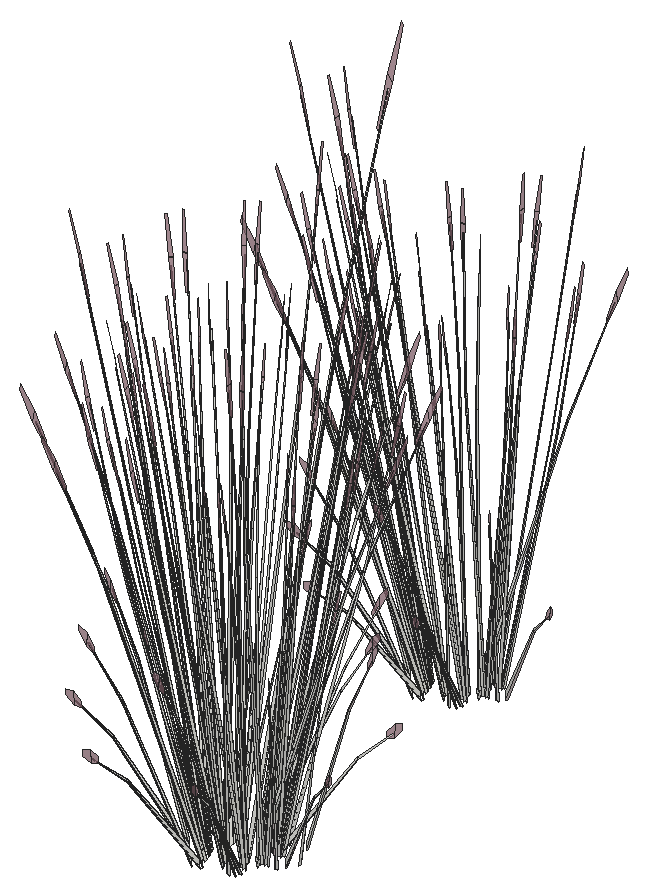
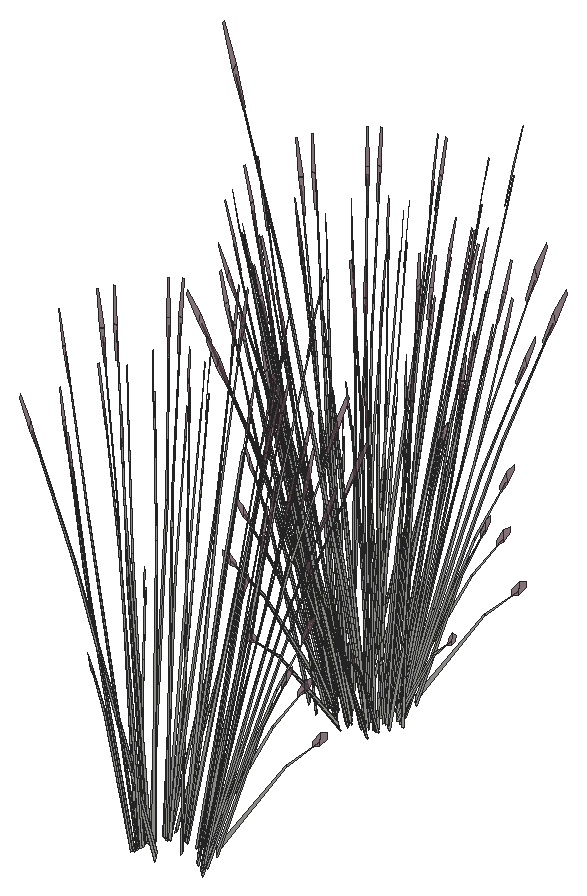
# SketchUp Ruby script. Lengths in inches.
U = 1.inch
M = Sketchup.active_model
def pt(a) = Geom::Point3d.new(a.map { |v| v * U })
def face(e, loops, mat)
  f = e.add_face(loops[0].map { |a| pt(a) })
  loops[1..].each { |l| e.add_face(l.map { |a| pt(a) }).erase! }
  f.material = f.back_material = mat if mat
  f
end
# faces: each face lists its corners as indices into pts; further lists are holes
def faces(e, pts, list, mat = nil) = list.each { |f| face(e, (f[0].is_a?(Array) ? f : [f]).map { |l| l.map { |i| pts[i] } }, mat) }
# xy, xz, yz: faces in a plane at the given z, y or x. An outline is a flat list of corners, or four numbers for a rectangle; further outlines are holes
def ring(l) = l.size == 4 ? [[l[0], l[1]], [l[2], l[1]], [l[2], l[3]], [l[0], l[3]]] : l.each_slice(2).to_a
def flat(e, list, mat, &to3) = list.each { |f| face(e, (f[0].is_a?(Array) ? f : [f]).map { |l| ring(l).map { |u, v| to3.(u, v) } }, mat) }
def xy(e, z, list, mat = nil) = flat(e, list, mat) { |x, y| [x, y, z] }
def xz(e, y, list, mat = nil) = flat(e, list, mat) { |x, z| [x, y, z] }
def yz(e, x, list, mat = nil) = flat(e, list, mat) { |y, z| [x, y, z] }
def lines(e, pts, list) = list.each { |a, b| e.add_line(pt(pts[a]), pt(pts[b])) }
# prism: a flat outline (further loops are holes) pulled along v
def prism(e, loops, v, mat = nil)
  f = face(e, loops, mat); d = Geom::Vector3d.new(v.map { |x| x * U })
  f.pushpull(f.normal.samedirection?(d) ? d.length : -d.length)
end
def box(e, o, s, mat = nil) = prism(e, [[o, [o[0] + s[0], o[1], o[2]], [o[0] + s[0], o[1] + s[1], o[2]], [o[0], o[1] + s[1], o[2]]]], [0, 0, s[2]], mat)
def at(x, y, z, deg = 0) = Geom::Transformation.translation(pt([x, y, z])) * Geom::Transformation.rotation(ORIGIN, Z_AXIS, deg.degrees)
def axes(o, x, y, z) = Geom::Transformation.new([*x, 0, *y, 0, *z, 0, *pt(o).to_a, 1])
def part(name) = M.definitions.add(name)
# library, detail: a bought-in or finely detailed component or shape, given as its bounding box
def library(name, o, s) = part(name).tap { |d| box(d.entities, o, s) }
def detail(e, o, s) = box(e.add_group.entities, o, s)
def put(e, d, t, mat = nil) = e.add_instance(d, t).tap { |i| i.material = mat if mat }
def group(e, t, mat = nil) = e.add_group.tap { |g| g.transformation = t; g.material = mat if mat }.entities
root = M.entities
M.materials.add("LightPink_Translucent").color = [144, 107, 117]
M.materials["LightPink_Translucent"].alpha = 0.75
c1 = part("blade")
p = [[2.15,0.21,22],[0,0.17,0],[0.09,0.45,0],[2.18,0.31,22],[2.29,0.31,22],[0.38,0.45,0],
  [2.48,0.24,33],[2.49,0.24,33],[2.48,0.22,33]]
faces(c1.entities,p,[[0,1,2,3],[4,5,2,3],[6,3,4,7],[8,0,3,6]])
c2 = part("seeds")
p = [[0.3,-0.1,1.38],[-0.01,-0.03,1.59],[-0.01,-0.03,0.03],[0.14,-0.07,-0.07],[0.29,-0.03,3],[0.15,0.01,3.11]]
faces(c2.entities,p,[[0,1,2,3],[1,0,4,5]],"LightPink_Translucent")
c3 = part("blade with seeds")
put(c3.entities,c1,at(0,0,0))
put(c3.entities,c2,axes([2.4,0.25,30.99],[1.5799,-0.05474,1.17369],[-0.12525,1.92788,0.29478],[-0.07173,-0.02425,1.56792]))
put(root,c3,axes([301.2,192.59,150.27],[0.09368,0.15143,1.44779],[-0.43286,0.12749,0.11706],[-0.09783,-0.23774,0.61892]))
put(root,c3,axes([301.91,191.58,150.98],[-0.06268,-0.06613,1.47793],[-0.4183,0.04193,-0.23373],[-0.06676,-0.15817,0.11853]))
put(root,c3,axes([303.79,192.39,150.98],[-0.00396,-0.09387,1.47793],[-0.33411,-0.2713,-0.23373],[0.05166,-0.16446,0.11853]))
put(root,c3,axes([302.39,192.375,150.82],[0.12355,-0.36271,-0.29918],[0.36044,0.10579,0.38624],[-0.03305,-0.14603,0.73904]))
put(root,c3,axes([302.66,192.85,150.27],[-0.0763,0.16212,1.44779],[-0.3201,-0.3355,0.11706],[0.1444,-0.2091,0.61892]))
put(root,c3,axes([303.7,192.06,150.98],[-0.04162,0.03603,1.49853],[-0.40776,-0.12155,-0.1416],[-0.01476,-0.15722,0.26519]))
put(root,c3,axes([301.49,191.37,150.98],[-0.00765,0.05653,1.49853],[-0.37706,0.20517,-0.1416],[-0.11096,-0.10488,0.26519]))
put(root,c3,axes([302.43,192.46,151],[0.4038,0.12331,0.40553],[-0.13808,0.40538,0.33437],[-0.02427,-0.15942,0.83914]))
put(root,c3,axes([302.55,192.6,151.25],[-0.40102,0.2196,-0.10273],[-0.19707,-0.38974,-0.57019],[-0.05291,-0.16424,0.8664]))
put(root,c3,axes([303.38,193.1,151.25],[-0.45039,-0.02337,-0.10273],[0.01231,-0.44247,-0.57019],[0.03129,-0.17041,0.8664]))
put(root,c3,axes([303.35,192.8125,150.82],[0.27728,-0.24833,-0.29918],[0.26248,0.28355,0.38624],[0.03994,-0.14407,0.73904]))
put(root,c3,axes([302.54,192.43,151],[0.30197,-0.1603,0.05432],[0.1478,0.29231,0.42765],[-0.02916,-0.12885,0.65209]))
put(root,c3,axes([301.35,192.51,150.82],[-0.06329,-0.37991,-0.29918],[0.36182,-0.10032,0.38624],[-0.09718,-0.10887,0.73904]))
put(root,c3,axes([301.51,192.47,151],[0.18625,-0.29962,0.05432],[0.26523,0.17444,0.42765],[-0.08575,-0.09606,0.65209]))
put(root,c3,axes([300.57,193.06,150.27],[0.15222,0.08126,1.44779],[-0.31502,0.34091,0.11706],[-0.19634,-0.15379,0.61892]))
put(root,c3,axes([302.43,192.76,151.27],[-0.12355,0.36271,0.29918],[-0.36044,-0.10579,-0.38624],[-0.03305,-0.14603,0.73904]))
put(root,c3,axes([303.35,192.91,151],[0.29182,0.32181,0.40553],[-0.3099,0.27755,0.33437],[0.05383,-0.15098,0.83914]))
put(root,c3,axes([301.59,192.44,151.59],[-0.2735,0.45217,-0.11506],[-0.39608,-0.2605,-0.63862],[-0.13768,-0.12775,0.97037]))
put(root,c3,axes([303.46,192.9375,151],[0.33677,0.02198,0.05432],[-0.00923,0.33185,0.42765],[0.03524,-0.12712,0.65209]))
put(root,c3,axes([303.21,193.16,151.27],[-0.27728,0.24833,0.29918],[-0.26248,-0.28355,-0.38624],[0.03994,-0.14407,0.73904]))
put(root,c3,axes([300.54,192.31,150.98],[-0.08817,-0.00333,1.47793],[-0.28072,0.33293,-0.23373],[-0.14978,-0.06803,0.11853]))
put(root,c3,axes([303.875,193.97,151.25],[-0.37908,-0.26007,-0.10273],[0.21839,-0.37663,-0.57019],[0.1071,-0.13092,0.8664]))
put(root,c3,axes([301.56,192.82,151.27],[0.06329,0.37991,0.29918],[-0.36182,0.10032,-0.38624],[-0.09718,-0.10887,0.73904]))
put(root,c3,axes([304.81,193.85,150.98],[-0.05353,-0.00358,1.49853],[-0.22227,-0.38383,-0.1416],[0.08926,-0.1262,0.26519]))
put(root,c3,axes([303.98,193.7,150.82],[0.35672,-0.06741,-0.29918],[0.09419,0.38534,0.38624],[0.10222,-0.1035,0.73904]))
put(root,c3,axes([300.63,193.0625,151],[0.02064,-0.35866,0.05432],[0.3116,0.00983,0.42765],[-0.11936,-0.03753,0.65209]))
put(root,c3,axes([300.51,193.17,150.82],[-0.23317,-0.29531,-0.29918],[0.26625,-0.27955,0.38624],[-0.13527,-0.04253,0.73904]))
put(root,c3,axes([303.6875,193.93,151.27],[-0.35672,0.06741,0.29918],[-0.09419,-0.38534,-0.38624],[0.10222,-0.1035,0.73904]))
put(root,c3,axes([304.01,193.87,151],[0.28133,0.19836,0.05432],[-0.16379,0.28248,0.42765],[0.0902,-0.09132,0.65209]))
put(root,c3,axes([303.93,193.79,151],[0.10163,0.43409,0.40553],[-0.39868,0.07534,0.33437],[0.1175,-0.10209,0.83914]))
put(root,c3,axes([305.01,194.3125,150.98],[0.05687,-0.07184,1.47793],[-0.07279,-0.44069,-0.23373],[0.14268,-0.08356,0.11853]))
put(root,c3,axes([300.2,192.59,150.98],[0.03038,0.04707,1.49853],[-0.14646,0.42312,-0.1416],[-0.14833,0.00306,0.26519]))
put(root,c3,axes([300.84,193.33,151.27],[0.23317,0.29531,0.29918],[-0.26625,0.27955,-0.38624],[-0.13527,-0.04253,0.73904]))
put(root,c3,axes([300.78,193.14,151.25],[-0.02194,0.47967,-0.10273],[-0.41546,-0.01311,-0.57019],[-0.16001,-0.03332,0.8664]))
put(root,c3,axes([303.89,194.98,151.25],[-0.20619,-0.42709,-0.10273],[0.36595,-0.20988,-0.57019],[0.15422,-0.05635,0.8664]))
put(root,c3,axes([300.25,193.8,150.27],[0.16998,-0.01068,1.44779],[-0.11276,0.46299,0.11706],[-0.24224,-0.02864,0.61892]))
put(root,c3,axes([303.75,194.85,151.27],[-0.34057,-0.13158,0.29918],[0.09933,-0.38387,-0.38624],[0.13712,-0.0352,0.73904]))
put(root,c3,axes([300.18,194.15,151],[0.11578,-0.43006,0.40553],[0.38064,0.14706,0.33437],[-0.14969,0.02584,0.83914]))
put(root,c3,axes([300.15,194.04,151],[-0.15051,-0.3216,0.05432],[0.27447,-0.15741,0.42765],[-0.12099,0.03106,0.65209]))
put(root,c3,axes([304.1,194.8125,150.82],[0.34057,0.13158,-0.29918],[-0.09933,0.38387,0.38624],[0.13712,-0.0352,0.73904]))
put(root,c3,axes([300.1,194.2,150.82],[-0.34057,-0.13158,-0.29918],[0.09933,-0.38387,0.38624],[-0.13712,0.0352,0.73904]))
put(root,c3,axes([303.18,194.34,150.27],[-0.16998,0.01068,1.44779],[0.11276,-0.46299,0.11706],[0.24224,0.02864,0.61892]))
put(root,c3,axes([304.05,194.97,151],[0.15051,0.3216,0.05432],[-0.27447,0.15741,0.42765],[0.12099,-0.03106,0.65209]))
put(root,c3,axes([304.03,194.86,151],[-0.11578,0.43006,0.40553],[-0.38064,-0.14706,0.33437],[0.14969,-0.02584,0.83914]))
put(root,c3,axes([300.46,194.16,151.27],[0.34057,0.13158,0.29918],[-0.09933,0.38387,-0.38624],[-0.13712,0.0352,0.73904]))
put(root,c3,axes([304.71,196.25,150.98],[-0.03706,-0.04129,1.49853],[0.08106,-0.44261,-0.1416],[0.14596,-0.02828,0.26519]))
put(root,c3,axes([299.89,194.45,150.98],[-0.06692,0.06124,1.47793],[0.00569,0.44742,-0.23373],[-0.15339,0.05818,0.11853]))
put(root,c3,axes([300.32,194.03,151.25],[0.20619,0.42709,-0.10273],[-0.36595,0.20988,-0.57019],[-0.15422,0.05635,0.8664]))
put(root,c3,axes([304.39,195.88,150.32],[-0.07843,-0.39649,-0.0295],[0.37072,-0.09115,-0.13375],[0.07742,0.02514,0.44114]))
put(root,c3,axes([303.43,195.87,151.25],[0.02194,-0.47967,-0.10273],[0.41546,0.01311,-0.57019],[0.16001,0.03332,0.8664]))
put(root,c3,axes([303.36,195.68,151.27],[-0.23317,-0.29531,0.29918],[0.26625,-0.27955,-0.38624],[0.13527,0.04253,0.73904]))
put(root,c3,axes([303.79,195.58,150.98],[0.08791,-0.00798,1.47793],[0.24113,-0.36643,-0.23373],[0.15637,0.04837,0.11853]))
put(root,c3,axes([300.27,195.22,151],[-0.10163,-0.43409,0.40553],[0.39868,-0.07534,0.33437],[-0.1175,0.10209,0.83914]))
put(root,c3,axes([300.19,195.14,151],[-0.28133,-0.19836,0.05432],[0.16379,-0.28248,0.42765],[-0.0902,0.09132,0.65209]))
put(root,c3,axes([300.32,194.62,150.27],[0.14219,-0.09977,1.44779],[0.11971,0.461,0.11706],[-0.22323,0.10419,0.61892]))
put(root,c3,axes([300.52,195.08,151.27],[0.35672,-0.06741,0.29918],[0.09419,0.38534,-0.38624],[-0.10222,0.1035,0.73904]))
put(root,c3,axes([299.14,194.91,150.98],[0.0523,0.01265,1.49853],[0.16179,0.41674,-0.1416],[-0.10706,0.10938,0.26519]))
put(root,c3,axes([303.69,195.84,150.82],[0.23317,0.29531,-0.29918],[-0.26625,0.27955,0.38624],[0.13527,0.04253,0.73904]))
put(root,c3,axes([303.57,195.95,151],[-0.02064,0.35866,0.05432],[-0.3116,-0.00983,0.42765],[0.11936,0.03753,0.65209]))
put(root,c3,axes([300.23,195.31,150.82],[-0.35672,0.06741,-0.29918],[-0.09419,-0.38534,0.38624],[-0.10222,0.1035,0.73904]))
put(root,c3,axes([303.6,195.83,151],[-0.30217,0.31079,0.40553],[-0.2606,-0.33005,0.33437],[0.14177,0.05733,0.83914]))
put(root,c3,axes([302.64,196.19,151.27],[-0.06329,-0.37991,0.29918],[0.36182,-0.10032,-0.38624],[0.09718,0.10887,0.73904]))
put(root,c3,axes([302.86,195.08,150.27],[-0.15222,-0.08126,1.44779],[0.31502,-0.34091,0.11706],[0.19634,0.15379,0.61892]))
put(root,c3,axes([302.88,194.01,150.78],[-0.35411,-0.24507,1.16821],[0.37391,-0.38156,0.50405],[0.11425,0.22994,1.12919]))
put(root,c3,axes([300.33,195.04,151.25],[0.37908,0.26007,-0.10273],[-0.21839,0.37663,-0.57019],[-0.1071,0.13092,0.8664]))
put(root,c3,axes([302.61,196.39,151.25],[0.2442,-0.40372,-0.10273],[0.35364,0.23259,-0.57019],[0.12293,0.11406,0.8664]))
put(root,c3,axes([300.84,194.93,150.27],[0.10236,-0.14492,1.44779],[0.25844,0.39118,0.11706],[-0.17726,0.17814,0.61892]))
put(root,c3,axes([301,195.85,151.27],[0.27728,-0.24833,0.29918],[0.26248,0.28355,-0.38624],[-0.03994,0.14407,0.73904]))
put(root,c3,axes([302.29,196.73,150.98],[0.00121,-0.0571,1.49853],[0.35119,-0.25193,-0.1416],[0.12199,0.08992,0.26519]))
put(root,c3,axes([300.75,196.07,151],[-0.33677,-0.02198,0.05432],[0.00923,-0.33185,0.42765],[-0.03524,0.12712,0.65209]))
put(root,c3,axes([300.85,196.1,151],[-0.29182,-0.32181,0.40553],[0.3099,-0.27755,0.33437],[-0.05383,0.15098,0.83914]))
put(root,c3,axes([301.78,196.25,151.27],[0.12355,-0.36271,0.29918],[0.36044,0.10579,-0.38624],[0.03305,0.14603,0.73904]))
put(root,c3,axes([302.7,196.54,151],[-0.18625,0.29962,0.05432],[-0.26523,-0.17444,0.42765],[0.08575,0.09606,0.65209]))
put(root,c3,axes([302.78,196.45,151],[-0.4076,0.10824,0.40553],[-0.07074,-0.4246,0.33437],[0.09586,0.12514,0.83914]))
put(root,c3,axes([300.77,195.28,150.27],[0.0763,-0.16212,1.44779],[0.3201,0.3355,0.11706],[-0.1444,0.2091,0.61892]))
put(root,c3,axes([301.66,196.58,151],[-0.30197,0.1603,0.05432],[-0.1478,-0.29231,0.42765],[0.02916,0.12885,0.65209]))
put(root,c3,axes([300.85,196.2,150.82],[-0.27728,0.24833,-0.29918],[-0.26248,-0.28355,0.38624],[-0.03994,0.14407,0.73904]))
put(root,c3,axes([299.9,196.125,150.98],[-0.01019,0.09334,1.47793],[0.28908,0.3247,-0.23373],[-0.07568,0.15355,0.11853]))
put(root,c3,axes([300.82,195.91,151.56],[0.45039,0.02337,-0.11403],[-0.01231,0.44247,-0.63292],[-0.03129,0.17041,0.9617]))
put(root,c3,axes([301.66,196.41,151.25],[0.40102,-0.2196,-0.10273],[0.19707,0.38974,-0.57019],[0.05291,0.16424,0.8664]))
put(root,c3,axes([302.23,195.55,150.27],[-0.09368,-0.15143,1.44779],[0.43286,-0.12749,0.11706],[0.09783,0.23774,0.61892]))
put(root,c3,axes([301.82,196.64,150.82],[-0.12355,0.36271,-0.29918],[-0.36044,-0.10579,0.38624],[0.03305,0.14603,0.73904]))
put(root,c3,axes([299.87,197.08,150.98],[0.04649,-0.02848,1.49853],[0.38427,0.18941,-0.1416],[-0.00903,0.15771,0.26519]))
put(root,c3,axes([301.46,195.625,150.27],[-0.01003,-0.18103,1.44779],[0.43473,0.12009,0.11706],[-0.02689,0.25798,0.61892]))
put(root,c3,axes([301.5625,197.28,150.98],[0.05195,0.07595,1.47793],[0.41921,0.02984,-0.23373],[0.04216,0.1675,0.11853]))
put(root,c3,axes([299.2,211.99,150.27],[0.09368,0.15143,1.44779],[-0.43286,0.12749,0.11706],[-0.09783,-0.23774,0.61892]))
put(root,c3,axes([299.91,210.99,150.98],[-0.06268,-0.06613,1.47793],[-0.4183,0.04193,-0.23373],[-0.06676,-0.15817,0.11853]))
put(root,c3,axes([301.79,211.8,150.98],[-0.00396,-0.09387,1.47793],[-0.33411,-0.2713,-0.23373],[0.05166,-0.16446,0.11853]))
put(root,c3,axes([300.39,211.78,150.82],[0.12355,-0.36271,-0.29918],[0.36044,0.10579,0.38624],[-0.03305,-0.14603,0.73904]))
put(root,c3,axes([300.66,212.26,150.27],[-0.0763,0.16212,1.44779],[-0.3201,-0.3355,0.11706],[0.1444,-0.2091,0.61892]))
put(root,c3,axes([301.7,211.46,150.98],[-0.04162,0.03603,1.49853],[-0.40776,-0.12155,-0.1416],[-0.01476,-0.15722,0.26519]))
put(root,c3,axes([299.49,210.77,150.98],[-0.00765,0.05653,1.49853],[-0.37706,0.20517,-0.1416],[-0.11096,-0.10488,0.26519]))
put(root,c3,axes([300.43,211.87,151],[0.4038,0.12331,0.40553],[-0.13808,0.40538,0.33437],[-0.02427,-0.15942,0.83914]))
put(root,c3,axes([300.55,212.01,151.25],[-0.40102,0.2196,-0.10273],[-0.19707,-0.38974,-0.57019],[-0.05291,-0.16424,0.8664]))
put(root,c3,axes([301.38,212.5,151.25],[-0.45039,-0.02337,-0.10273],[0.01231,-0.44247,-0.57019],[0.03129,-0.17041,0.8664]))
put(root,c3,axes([301.35,212.22,150.82],[0.27728,-0.24833,-0.29918],[0.26248,0.28355,0.38624],[0.03994,-0.14407,0.73904]))
put(root,c3,axes([300.54,211.84,151],[0.30197,-0.1603,0.05432],[0.1478,0.29231,0.42765],[-0.02916,-0.12885,0.65209]))
put(root,c3,axes([299.35,211.91,150.82],[-0.06329,-0.37991,-0.29918],[0.36182,-0.10032,0.38624],[-0.09718,-0.10887,0.73904]))
put(root,c3,axes([299.51,211.88,151],[0.18625,-0.29962,0.05432],[0.26523,0.17444,0.42765],[-0.08575,-0.09606,0.65209]))
put(root,c3,axes([298.57,212.47,150.27],[0.15222,0.08126,1.44779],[-0.31502,0.34091,0.11706],[-0.19634,-0.15379,0.61892]))
put(root,c3,axes([300.43,212.16,151.27],[-0.12355,0.36271,0.29918],[-0.36044,-0.10579,-0.38624],[-0.03305,-0.14603,0.73904]))
put(root,c3,axes([301.35,212.32,151],[0.29182,0.32181,0.40553],[-0.3099,0.27755,0.33437],[0.05383,-0.15098,0.83914]))
put(root,c3,axes([299.59,211.85,151.59],[-0.2735,0.45217,-0.11506],[-0.39608,-0.2605,-0.63862],[-0.13768,-0.12775,0.97037]))
put(root,c3,axes([301.46,212.35,151],[0.33677,0.02198,0.05432],[-0.00923,0.33185,0.42765],[0.03524,-0.12712,0.65209]))
put(root,c3,axes([301.21,212.57,151.27],[-0.27728,0.24833,0.29918],[-0.26248,-0.28355,-0.38624],[0.03994,-0.14407,0.73904]))
put(root,c3,axes([298.54,211.72,150.98],[-0.08817,-0.00333,1.47793],[-0.28072,0.33293,-0.23373],[-0.14978,-0.06803,0.11853]))
put(root,c3,axes([301.875,213.375,151.25],[-0.37908,-0.26007,-0.10273],[0.21839,-0.37663,-0.57019],[0.1071,-0.13092,0.8664]))
put(root,c3,axes([299.56,212.22,151.27],[0.06329,0.37991,0.29918],[-0.36182,0.10032,-0.38624],[-0.09718,-0.10887,0.73904]))
put(root,c3,axes([302.81,213.26,150.98],[-0.05353,-0.00358,1.49853],[-0.22227,-0.38383,-0.1416],[0.08926,-0.1262,0.26519]))
put(root,c3,axes([301.98,213.11,150.82],[0.35672,-0.06741,-0.29918],[0.09419,0.38534,0.38624],[0.10222,-0.1035,0.73904]))
put(root,c3,axes([298.63,212.47,151],[0.02064,-0.35866,0.05432],[0.3116,0.00983,0.42765],[-0.11936,-0.03753,0.65209]))
put(root,c3,axes([298.51,212.58,150.82],[-0.23317,-0.29531,-0.29918],[0.26625,-0.27955,0.38624],[-0.13527,-0.04253,0.73904]))
put(root,c3,axes([301.6875,213.34,151.27],[-0.35672,0.06741,0.29918],[-0.09419,-0.38534,-0.38624],[0.10222,-0.1035,0.73904]))
put(root,c3,axes([302.01,213.28,151],[0.28133,0.19836,0.05432],[-0.16379,0.28248,0.42765],[0.0902,-0.09132,0.65209]))
put(root,c3,axes([301.93,213.2,151],[0.10163,0.43409,0.40553],[-0.39868,0.07534,0.33437],[0.1175,-0.10209,0.83914]))
put(root,c3,axes([303.01,213.72,150.98],[0.05687,-0.07184,1.47793],[-0.07279,-0.44069,-0.23373],[0.14268,-0.08356,0.11853]))
put(root,c3,axes([298.2,212,150.98],[0.03038,0.04707,1.49853],[-0.14646,0.42312,-0.1416],[-0.14833,0.00306,0.26519]))
put(root,c3,axes([298.84,212.74,151.27],[0.23317,0.29531,0.29918],[-0.26625,0.27955,-0.38624],[-0.13527,-0.04253,0.73904]))
put(root,c3,axes([298.78,212.55,151.25],[-0.02194,0.47967,-0.10273],[-0.41546,-0.01311,-0.57019],[-0.16001,-0.03332,0.8664]))
put(root,c3,axes([301.89,214.39,151.25],[-0.20619,-0.42709,-0.10273],[0.36595,-0.20988,-0.57019],[0.15422,-0.05635,0.8664]))
put(root,c3,axes([298.25,213.21,150.27],[0.16998,-0.01068,1.44779],[-0.11276,0.46299,0.11706],[-0.24224,-0.02864,0.61892]))
put(root,c3,axes([301.75,214.26,151.27],[-0.34057,-0.13158,0.29918],[0.09933,-0.38387,-0.38624],[0.13712,-0.0352,0.73904]))
put(root,c3,axes([298.18,213.56,151],[0.11578,-0.43006,0.40553],[0.38064,0.14706,0.33437],[-0.14969,0.02584,0.83914]))
put(root,c3,axes([298.15,213.45,151],[-0.15051,-0.3216,0.05432],[0.27447,-0.15741,0.42765],[-0.12099,0.03106,0.65209]))
put(root,c3,axes([302.1,214.22,150.82],[0.34057,0.13158,-0.29918],[-0.09933,0.38387,0.38624],[0.13712,-0.0352,0.73904]))
put(root,c3,axes([298.1,213.61,150.82],[-0.34057,-0.13158,-0.29918],[0.09933,-0.38387,0.38624],[-0.13712,0.0352,0.73904]))
put(root,c3,axes([301.18,213.74,150.27],[-0.16998,0.01068,1.44779],[0.11276,-0.46299,0.11706],[0.24224,0.02864,0.61892]))
put(root,c3,axes([302.05,214.38,151],[0.15051,0.3216,0.05432],[-0.27447,0.15741,0.42765],[0.12099,-0.03106,0.65209]))
put(root,c3,axes([302.03,214.27,151],[-0.11578,0.43006,0.40553],[-0.38064,-0.14706,0.33437],[0.14969,-0.02584,0.83914]))
